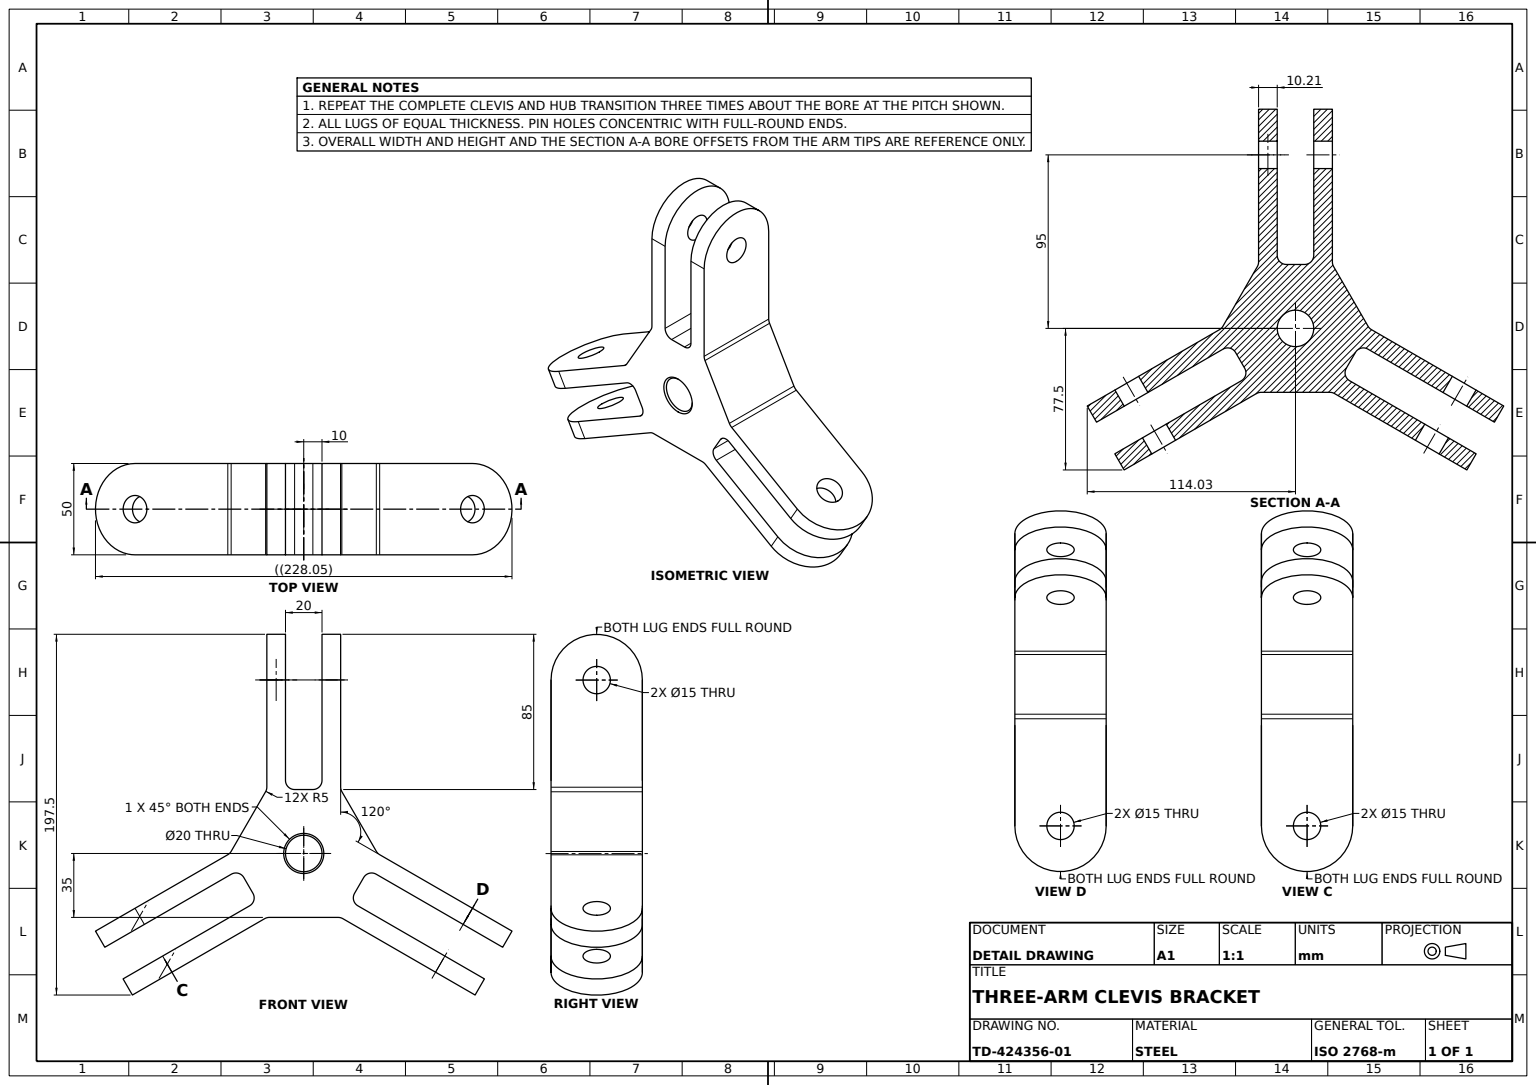
solid
v1 (-39.641016,-25,11.339746)
v2 (-39.641016,25,11.339746)
e1 v1 v2 LINE
v3 (-87.272413,25,38.839746)
e2 v3 v2 LINE
v4 (-87.272413,-25,38.839746)
e3 v3 v4 CIRCLE(AX(P(-87.272413,0,38.839746),D(0.5,0,0.866025404),D(-0.866025404,0,0.5)),25)
e4 v4 v1 LINE
v5 (-80.777223,0,35.089746)
v6 (-93.767604,0,42.589746)
e5 v5 v6 CIRCLE(AX(P(-87.272413,0,38.839746),D(-0.5,0,-0.866025404),D(-0.866025404,0,0.5)),7.5)
e6 v6 v5 CIRCLE(AX(P(-87.272413,0,38.839746),D(-0.5,0,-0.866025404),D(-0.866025404,0,0.5)),7.5)
face PLANE(AX(P(-108.923048,25,51.339746),D(-0.5,0,-0.866025404),D(-0.866025404,0,0.5))) rev [e1 -e2 e3 e4] [e5 e6]
v7 (39.744646,25,-1.160254)
v8 (20.877132,25,-33.839746)
e7 v7 v8 LINE
v9 (39.744646,-25,-1.160254)
e8 v7 v9 LINE
v10 (20.877132,-25,-33.839746)
e9 v9 v10 LINE
e10 v10 v8 LINE
face PLANE(AX(P(40.414519,25,0),D(-0.866025404,0,0.5),D(0.5,0,0.866025404))) rev [-e7 e8 e9 e10]
v11 (93.767604,0,42.589746)
v12 (80.777223,0,35.089746)
e11 v11 v12 CIRCLE(AX(P(87.272413,0,38.839746),D(0.5,0,-0.866025404),D(-0.866025404,0,-0.5)),7.5)
v13 (98.871234,0,33.75)
e12 v13 v11 LINE
v14 (85.880853,0,26.25)
e13 v13 v14 CIRCLE(AX(P(92.376043,0,30),D(0.5,0,-0.866025404),D(0.866025404,0,0.5)),7.5)
e14 v14 v12 LINE
face CYL(AX(P(102.982645,0,11.628827),D(-0.5,0,0.866025404),D(0.866025404,0,0.5)),7.5) rev [-e11 -e12 e13 e14]
v15 (0,-24,10)
v16 (0,-24,-10)
e15 v15 v16 CIRCLE(AX(P(0,-24,0),D(0,-1,0),D(0,0,-1)),10)
v17 (0,24,-10)
e16 v17 v16 LINE
v18 (0,24,10)
e17 v17 v18 CIRCLE(AX(P(0,24,0),D(0,1,0),D(0,0,-1)),10)
e18 v18 v15 LINE
face CYL(AX(P(0,53.284271,0),D(0,-1,0),D(0,0,-1)),10) rev [e15 -e16 e17 e18]
v19 (-85.880853,0,26.25)
v20 (-98.871234,0,33.75)
e19 v19 v20 CIRCLE(AX(P(-92.376043,0,30),D(-0.5,0,-0.866025404),D(0.866025404,0,-0.5)),7.5)
e20 v20 v6 LINE
e21 v19 v5 LINE
face CYL(AX(P(-102.982645,0,11.628827),D(0.5,0,0.866025404),D(0.866025404,0,-0.5)),7.5) rev [e19 e20 -e5 -e21]
v21 (-70.777223,0,52.410254)
v22 (-83.767604,0,59.910254)
e22 v21 v22 CIRCLE(AX(P(-77.272413,0,56.160254),D(0.5,0,0.866025404),D(0.866025404,0,-0.5)),7.5)
v23 (-65.673593,0,61.25)
e23 v21 v23 LINE
v24 (-78.663974,0,68.75)
e24 v23 v24 CIRCLE(AX(P(-72.168784,0,65),D(0.5,0,0.866025404),D(0.866025404,0,-0.5)),7.5)
e25 v22 v24 LINE
face CYL(AX(P(-102.982645,0,11.628827),D(0.5,0,0.866025404),D(0.866025404,0,-0.5)),7.5) rev [-e22 e23 e24 -e25]
v25 (78.663974,0,68.75)
v26 (65.673593,0,61.25)
e26 v25 v26 CIRCLE(AX(P(72.168784,0,65),D(-0.5,0,0.866025404),D(0.866025404,0,0.5)),7.5)
e27 v26 v25 CIRCLE(AX(P(72.168784,0,65),D(-0.5,0,0.866025404),D(0.866025404,0,0.5)),7.5)
v27 (21.367513,-25,35.669873)
v28 (72.168784,-25,65)
e28 v27 v28 LINE
v29 (72.168784,25,65)
e29 v28 v29 CIRCLE(AX(P(72.168784,0,65),D(-0.5,0,0.866025404),D(-0.866025404,0,-0.5)),25)
v30 (21.367513,25,35.669873)
e30 v30 v29 LINE
e31 v30 v27 LINE
face PLANE(AX(P(93.819419,25,77.5),D(0.5,0,-0.866025404),D(-0.866025404,0,-0.5))) rev [-e26 -e27] [e28 e29 -e30 e31]
v31 (92.376043,25,30)
v32 (41.574773,25,0.669873)
e32 v31 v32 LINE
v33 (92.376043,-25,30)
e33 v31 v33 CIRCLE(AX(P(92.376043,0,30),D(0.5,0,-0.866025404),D(0.866025404,0,0.5)),25)
v34 (41.574773,-25,0.669873)
e34 v33 v34 LINE
e35 v34 v32 LINE
e36 v14 v13 CIRCLE(AX(P(92.376043,0,30),D(0.5,0,-0.866025404),D(0.866025404,0,0.5)),7.5)
face PLANE(AX(P(40.414519,25,0),D(-0.5,0,0.866025404),D(0.866025404,0,0.5))) rev [-e32 e33 e34 e35] [-e13 -e36]
v35 (-77.272413,25,56.160254)
v36 (-72.168784,25,65)
e37 v35 v36 LINE
v37 (-77.272413,-25,56.160254)
e38 v37 v35 CIRCLE(AX(P(-77.272413,0,56.160254),D(-0.5,0,-0.866025404),D(0.866025404,0,-0.5)),25)
v38 (-72.168784,-25,65)
e39 v38 v37 LINE
e40 v36 v38 CIRCLE(AX(P(-72.168784,0,65),D(0.5,0,0.866025404),D(-0.866025404,0,0.5)),25)
face CYL(AX(P(-77.272413,0,56.160254),D(0.5,0,0.866025404),D(0.866025404,0,-0.5)),25) [-e37 -e38 -e39 -e40]
v39 (29.641016,25,28.660254)
v40 (27.810889,25,21.830127)
e41 v39 v40 CIRCLE(AX(P(32.141016,25,24.330127),D(0,-1,0),D(0,0,-1)),5)
v41 (29.641016,-25,28.660254)
e42 v41 v39 LINE
v42 (27.810889,-25,21.830127)
e43 v42 v41 CIRCLE(AX(P(32.141016,-25,24.330127),D(0,1,0),D(0,0,-1)),5)
e44 v40 v42 LINE
face CYL(AX(P(32.141016,25,24.330127),D(0,1,0),D(0,0,1)),5) rev [-e41 -e42 -e43 -e44]
e45 v12 v11 CIRCLE(AX(P(87.272413,0,38.839746),D(0.5,0,-0.866025404),D(-0.866025404,0,-0.5)),7.5)
v43 (87.272413,-25,38.839746)
v44 (87.272413,25,38.839746)
e46 v43 v44 CIRCLE(AX(P(87.272413,0,38.839746),D(-0.5,0,0.866025404),D(-0.866025404,0,-0.5)),25)
v45 (39.641016,25,11.339746)
e47 v45 v44 LINE
v46 (39.641016,-25,11.339746)
e48 v45 v46 LINE
e49 v46 v43 LINE
face PLANE(AX(P(108.923048,25,51.339746),D(0.5,0,-0.866025404),D(-0.866025404,0,-0.5))) rev [e45 e11] [e46 -e47 e48 e49]
v47 (-18.867513,25,35)
v48 (-18.867513,-25,35)
e50 v47 v48 LINE
v49 (-21.367513,25,35.669873)
e51 v49 v47 CIRCLE(AX(P(-18.867513,25,40),D(0,-1,0),D(0,0,-1)),5)
v50 (-21.367513,-25,35.669873)
e52 v50 v49 LINE
e53 v48 v50 CIRCLE(AX(P(-18.867513,-25,40),D(0,1,0),D(0,0,-1)),5)
face CYL(AX(P(-18.867513,25,40),D(0,1,0),D(0,0,1)),5) rev [-e50 -e51 -e52 -e53]
v51 (77.272413,25,56.160254)
e54 v29 v51 LINE
v52 (77.272413,-25,56.160254)
e55 v52 v28 LINE
e56 v51 v52 CIRCLE(AX(P(77.272413,0,56.160254),D(0.5,0,-0.866025404),D(0.866025404,0,0.5)),25)
face CYL(AX(P(72.168784,0,65),D(0.5,0,-0.866025404),D(-0.866025404,0,-0.5)),25) [-e54 -e29 -e55 -e56]
v53 (-10,0,-87.5)
v54 (-20.207259,0,-87.5)
e57 v53 v54 LINE
v55 (-10,0,-102.5)
e58 v55 v53 CIRCLE(AX(P(-10,0,-95),D(-1,0,0),D(0,0,1)),7.5)
v56 (-20.207259,0,-102.5)
e59 v55 v56 LINE
e60 v56 v54 CIRCLE(AX(P(-20.207259,0,-95),D(-1,0,0),D(0,0,1)),7.5)
face CYL(AX(P(41.420463,0,-95),D(-1,0,0),D(0,0,1)),7.5) rev [-e57 -e58 e59 e60]
face CYL(AX(P(102.982645,0,11.628827),D(-0.5,0,0.866025404),D(0.866025404,0,0.5)),7.5) rev [-e45 -e14 e36 e12]
v57 (20.207259,0,-87.5)
v58 (20.207259,0,-102.5)
e61 v57 v58 CIRCLE(AX(P(20.207259,0,-95),D(1,0,0),D(0,0,1)),7.5)
e62 v58 v57 CIRCLE(AX(P(20.207259,0,-95),D(1,0,0),D(0,0,1)),7.5)
v59 (20.207259,-25,-95)
v60 (20.207259,25,-95)
e63 v59 v60 CIRCLE(AX(P(20.207259,0,-95),D(1,0,0),D(0,0,1)),25)
v61 (20.207259,25,-36.339746)
e64 v61 v60 LINE
v62 (20.207259,-25,-36.339746)
e65 v61 v62 LINE
e66 v62 v59 LINE
face PLANE(AX(P(20.207259,25,-120),D(-1,0,0),D(0,0,1))) rev [-e61 -e62] [e63 -e64 e65 e66]
v63 (-20.207259,25,-95)
v64 (-20.207259,25,-36.339746)
e67 v63 v64 LINE
v65 (-20.207259,-25,-95)
e68 v63 v65 CIRCLE(AX(P(-20.207259,0,-95),D(-1,0,0),D(0,0,-1)),25)
v66 (-20.207259,-25,-36.339746)
e69 v65 v66 LINE
e70 v66 v64 LINE
e71 v54 v56 CIRCLE(AX(P(-20.207259,0,-95),D(-1,0,0),D(0,0,1)),7.5)
face PLANE(AX(P(-20.207259,25,-35),D(1,0,0),D(0,0,-1))) rev [-e67 e68 e69 e70] [-e71 -e60]
e72 v38 v50 LINE
e73 v36 v49 LINE
e74 v24 v23 CIRCLE(AX(P(-72.168784,0,65),D(0.5,0,0.866025404),D(0.866025404,0,-0.5)),7.5)
face PLANE(AX(P(-20.207259,25,35),D(-0.5,0,-0.866025404),D(-0.866025404,0,0.5))) rev [e40 e72 e52 -e73] [-e24 -e74]
e75 v53 v55 CIRCLE(AX(P(-10,0,-95),D(-1,0,0),D(0,0,1)),7.5)
v67 (-10,25,-40)
v68 (-10,25,-95)
e76 v67 v68 LINE
v69 (-10,-25,-40)
e77 v67 v69 LINE
v70 (-10,-25,-95)
e78 v69 v70 LINE
e79 v70 v68 CIRCLE(AX(P(-10,0,-95),D(1,0,0),D(0,0,1)),25)
face PLANE(AX(P(-10,25,-120),D(-1,0,0),D(0,0,1))) rev [e58 e75] [-e76 e77 e78 e79]
v71 (-41.574773,25,0.669873)
v72 (-92.376043,25,30)
e80 v71 v72 LINE
v73 (-41.574773,-25,0.669873)
e81 v71 v73 LINE
v74 (-92.376043,-25,30)
e82 v73 v74 LINE
e83 v74 v72 CIRCLE(AX(P(-92.376043,0,30),D(-0.5,0,-0.866025404),D(0.866025404,0,-0.5)),25)
e84 v20 v19 CIRCLE(AX(P(-92.376043,0,30),D(-0.5,0,-0.866025404),D(0.866025404,0,-0.5)),7.5)
face PLANE(AX(P(-114.026678,25,42.5),D(0.5,0,0.866025404),D(0.866025404,0,-0.5))) rev [-e80 e81 e82 e83] [-e84 -e19]
v75 (70.777223,0,52.410254)
e85 v75 v26 LINE
v76 (83.767604,0,59.910254)
e86 v76 v25 LINE
e87 v75 v76 CIRCLE(AX(P(77.272413,0,56.160254),D(-0.5,0,0.866025404),D(0.866025404,0,0.5)),7.5)
face CYL(AX(P(102.982645,0,11.628827),D(-0.5,0,0.866025404),D(0.866025404,0,0.5)),7.5) rev [e85 e27 -e86 -e87]
e88 v76 v75 CIRCLE(AX(P(77.272413,0,56.160254),D(-0.5,0,0.866025404),D(0.866025404,0,0.5)),7.5)
e89 v51 v39 LINE
e90 v52 v41 LINE
face PLANE(AX(P(98.923048,25,68.660254),D(-0.5,0,0.866025404),D(0.866025404,0,0.5))) rev [e87 e88] [e42 -e89 e56 e90]
v77 (10,0,-87.5)
v78 (10,0,-102.5)
e91 v77 v78 CIRCLE(AX(P(10,0,-95),D(1,0,0),D(0,0,-1)),7.5)
e92 v57 v77 LINE
e93 v58 v78 LINE
face CYL(AX(P(41.420463,0,-95),D(-1,0,0),D(0,0,1)),7.5) rev [-e91 -e92 e61 e93]
e94 v68 v63 LINE
e95 v65 v70 LINE
face CYL(AX(P(-10,0,-95),D(-1,0,0),D(0,0,1)),25) [-e68 -e94 -e79 -e95]
v79 (0,-25,11)
e96 v15 v79 LINE
v80 (0,-25,-11)
e97 v80 v79 CIRCLE(AX(P(0,-25,0),D(0,1,0),D(0,0,-1)),11)
e98 v16 v80 LINE
face CONE(AX(P(0,-24,0),D(0,-1,0),D(0,0,-1)),10,0.785398163) rev [e96 -e97 -e98 -e15]
v81 (18.867513,25,35)
e99 v81 v30 CIRCLE(AX(P(18.867513,25,40),D(0,-1,0),D(0,0,-1)),5)
v82 (32.810889,25,13.169873)
e100 v40 v82 LINE
e101 v82 v45 CIRCLE(AX(P(37.141016,25,15.669873),D(0,-1,0),D(0,0,-1)),5)
e102 v44 v31 LINE
e103 v32 v7 CIRCLE(AX(P(44.074773,25,-3.660254),D(0,-1,0),D(0,0,-1)),5)
e104 v8 v61 CIRCLE(AX(P(25.207259,25,-36.339746),D(0,-1,0),D(0,0,-1)),5)
v83 (10,25,-95)
e105 v60 v83 LINE
v84 (10,25,-40)
e106 v83 v84 LINE
v85 (5,25,-35)
e107 v84 v85 CIRCLE(AX(P(5,25,-40),D(0,-1,0),D(0,0,-1)),5)
v86 (-5,25,-35)
e108 v85 v86 LINE
e109 v86 v67 CIRCLE(AX(P(-5,25,-40),D(0,-1,0),D(0,0,-1)),5)
v87 (-20.877132,25,-33.839746)
e110 v64 v87 CIRCLE(AX(P(-25.207259,25,-36.339746),D(0,-1,0),D(0,0,-1)),5)
v88 (-39.744646,25,-1.160254)
e111 v87 v88 LINE
e112 v88 v71 CIRCLE(AX(P(-44.074773,25,-3.660254),D(0,-1,0),D(0,0,-1)),5)
e113 v72 v3 LINE
v89 (-32.810889,25,13.169873)
e114 v2 v89 CIRCLE(AX(P(-37.141016,25,15.669873),D(0,-1,0),D(0,0,-1)),5)
v90 (-27.810889,25,21.830127)
e115 v89 v90 LINE
v91 (-29.641016,25,28.660254)
e116 v90 v91 CIRCLE(AX(P(-32.141016,25,24.330127),D(0,-1,0),D(0,0,-1)),5)
e117 v91 v35 LINE
e118 v47 v81 LINE
v92 (0,25,-11)
v93 (0,25,11)
e119 v92 v93 CIRCLE(AX(P(0,25,0),D(0,-1,0),D(0,0,-1)),11)
e120 v93 v92 CIRCLE(AX(P(0,25,0),D(0,-1,0),D(0,0,-1)),11)
face PLANE(AX(P(0,25,0),D(0,-1,0),D(0,0,-1))) rev [e99 e30 e54 e89 e41 e100 e101 e47 e102 e32 e103 e7 e104 e64 e105 e106 e107 e108 e109 e76 e94 e67 e110 e111 e112 e80 e113 e2 e114 e115 e116 e117 e37 e73 e51 e118] [e119 e120]
v94 (-27.810889,-25,21.830127)
e121 v94 v90 LINE
v95 (-29.641016,-25,28.660254)
e122 v95 v94 CIRCLE(AX(P(-32.141016,-25,24.330127),D(0,1,0),D(0,0,-1)),5)
e123 v91 v95 LINE
face CYL(AX(P(-32.141016,25,24.330127),D(0,1,0),D(0,0,1)),5) rev [-e116 -e121 -e122 -e123]
v96 (-39.744646,-25,-1.160254)
e124 v96 v88 LINE
e125 v73 v96 CIRCLE(AX(P(-44.074773,-25,-3.660254),D(0,1,0),D(0,0,-1)),5)
face CYL(AX(P(-44.074773,25,-3.660254),D(0,1,0),D(0,0,1)),5) rev [-e112 -e124 -e125 -e81]
v97 (18.867513,-25,35)
e126 v97 v81 LINE
e127 v27 v97 CIRCLE(AX(P(18.867513,-25,40),D(0,1,0),D(0,0,-1)),5)
face CYL(AX(P(18.867513,25,40),D(0,1,0),D(0,0,1)),5) rev [-e126 -e127 -e31 -e99]
v98 (-20.877132,-25,-33.839746)
e128 v98 v66 CIRCLE(AX(P(-25.207259,-25,-36.339746),D(0,1,0),D(0,0,-1)),5)
e129 v87 v98 LINE
face CYL(AX(P(-25.207259,25,-36.339746),D(0,1,0),D(0,0,1)),5) rev [-e110 -e70 -e128 -e129]
e130 v22 v21 CIRCLE(AX(P(-77.272413,0,56.160254),D(0.5,0,0.866025404),D(0.866025404,0,-0.5)),7.5)
e131 v95 v37 LINE
face PLANE(AX(P(-98.923048,25,68.660254),D(0.5,0,0.866025404),D(0.866025404,0,-0.5))) rev [e22 e130] [e123 e131 e38 -e117]
face CYL(AX(P(41.420463,0,-95),D(-1,0,0),D(0,0,1)),7.5) rev [-e75 e57 e71 -e59]
e132 v16 v15 CIRCLE(AX(P(0,-24,0),D(0,-1,0),D(0,0,-1)),10)
e133 v18 v17 CIRCLE(AX(P(0,24,0),D(0,1,0),D(0,0,-1)),10)
face CYL(AX(P(0,53.284271,0),D(0,-1,0),D(0,0,-1)),10) rev [e132 -e18 e133 e16]
v99 (10,-25,-95)
e134 v99 v59 LINE
e135 v62 v10 CIRCLE(AX(P(25.207259,-25,-36.339746),D(0,1,0),D(0,0,-1)),5)
e136 v9 v34 CIRCLE(AX(P(44.074773,-25,-3.660254),D(0,1,0),D(0,0,-1)),5)
e137 v33 v43 LINE
v100 (32.810889,-25,13.169873)
e138 v46 v100 CIRCLE(AX(P(37.141016,-25,15.669873),D(0,1,0),D(0,0,-1)),5)
e139 v42 v100 LINE
e140 v48 v97 LINE
v101 (-32.810889,-25,13.169873)
e141 v101 v94 LINE
e142 v101 v1 CIRCLE(AX(P(-37.141016,-25,15.669873),D(0,1,0),D(0,0,-1)),5)
e143 v4 v74 LINE
e144 v98 v96 LINE
v102 (-5,-25,-35)
e145 v69 v102 CIRCLE(AX(P(-5,-25,-40),D(0,1,0),D(0,0,-1)),5)
v103 (5,-25,-35)
e146 v103 v102 LINE
v104 (10,-25,-40)
e147 v103 v104 CIRCLE(AX(P(5,-25,-40),D(0,1,0),D(0,0,-1)),5)
e148 v99 v104 LINE
e149 v79 v80 CIRCLE(AX(P(0,-25,0),D(0,1,0),D(0,0,-1)),11)
face PLANE(AX(P(0,-25,0),D(0,-1,0),D(0,0,-1))) [e134 -e66 e135 -e9 e136 -e34 e137 -e49 e138 -e139 e43 -e90 e55 -e28 e127 -e140 e53 -e72 e39 -e131 e122 -e141 e142 -e4 e143 -e82 e125 -e144 e128 -e69 e95 -e78 e145 -e146 e147 -e148] [e149 e97]
face CYL(AX(P(44.074773,25,-3.660254),D(0,1,0),D(0,0,1)),5) rev [-e35 -e136 -e8 -e103]
e150 v78 v77 CIRCLE(AX(P(10,0,-95),D(1,0,0),D(0,0,-1)),7.5)
e151 v83 v99 CIRCLE(AX(P(10,0,-95),D(-1,0,0),D(0,0,-1)),25)
e152 v104 v84 LINE
face PLANE(AX(P(10,25,-120),D(1,0,0),D(0,0,-1))) rev [e91 e150] [e151 e148 e152 -e106]
face CYL(AX(P(102.982645,0,11.628827),D(-0.5,0,0.866025404),D(0.866025404,0,0.5)),7.5) rev [-e88 e86 e26 -e85]
e153 v85 v103 LINE
face CYL(AX(P(5,25,-40),D(0,1,0),D(0,0,1)),5) rev [-e153 -e107 -e152 -e147]
face CYL(AX(P(25.207259,25,-36.339746),D(0,1,0),D(0,0,1)),5) rev [-e10 -e135 -e65 -e104]
face PLANE(AX(P(-20.207259,25,35),D(0,0,-1),D(-1,0,0))) rev [e50 e140 e126 -e118]
e154 v102 v86 LINE
face PLANE(AX(P(-10,25,-35),D(0,0,1),D(1,0,0))) rev [-e108 e153 e146 e154]
e155 v17 v92 LINE
e156 v18 v93 LINE
face CONE(AX(P(0,24,0),D(0,1,0),D(0,0,1)),10,0.785398163) rev [-e17 e155 -e120 -e156]
face PLANE(AX(P(-20.207259,25,-35),D(0.866025404,0,0.5),D(0.5,0,-0.866025404))) rev [-e111 e129 e144 e124]
face CYL(AX(P(-92.376043,0,30),D(0.5,0,0.866025404),D(0.866025404,0,-0.5)),25) [-e143 -e3 -e113 -e83]
face CYL(AX(P(41.420463,0,-95),D(-1,0,0),D(0,0,1)),7.5) rev [-e150 -e93 e62 e92]
face CYL(AX(P(-102.982645,0,11.628827),D(0.5,0,0.866025404),D(0.866025404,0,-0.5)),7.5) rev [-e130 e25 e74 -e23]
e157 v100 v82 LINE
face PLANE(AX(P(25.310889,25,26.160254),D(-0.866025404,0,-0.5),D(-0.5,0,0.866025404))) rev [e139 e157 -e100 e44]
face CYL(AX(P(-5,25,-40),D(0,1,0),D(0,0,1)),5) rev [-e145 -e77 -e109 -e154]
face CYL(AX(P(87.272413,0,38.839746),D(0.5,0,-0.866025404),D(-0.866025404,0,-0.5)),25) [-e33 -e102 -e46 -e137]
e158 v89 v101 LINE
face CYL(AX(P(-37.141016,25,15.669873),D(0,1,0),D(0,0,1)),5) rev [-e142 -e158 -e114 -e1]
face CYL(AX(P(37.141016,25,15.669873),D(0,1,0),D(0,0,1)),5) rev [-e157 -e138 -e48 -e101]
face CONE(AX(P(0,-24,0),D(0,-1,0),D(0,0,-1)),10,0.785398163) rev [e98 -e149 -e96 -e132]
face PLANE(AX(P(-35.310889,25,8.839746),D(0.866025404,0,-0.5),D(-0.5,0,-0.866025404))) rev [e158 e141 e121 -e115]
face CYL(AX(P(20.207259,0,-95),D(-1,0,0),D(0,0,1)),25) [-e63 -e134 -e151 -e105]
face CYL(AX(P(-102.982645,0,11.628827),D(0.5,0,0.866025404),D(0.866025404,0,-0.5)),7.5) rev [e21 -e6 -e20 e84]
face CONE(AX(P(0,24,0),D(0,1,0),D(0,0,1)),10,0.785398163) rev [-e119 -e155 -e133 e156]
